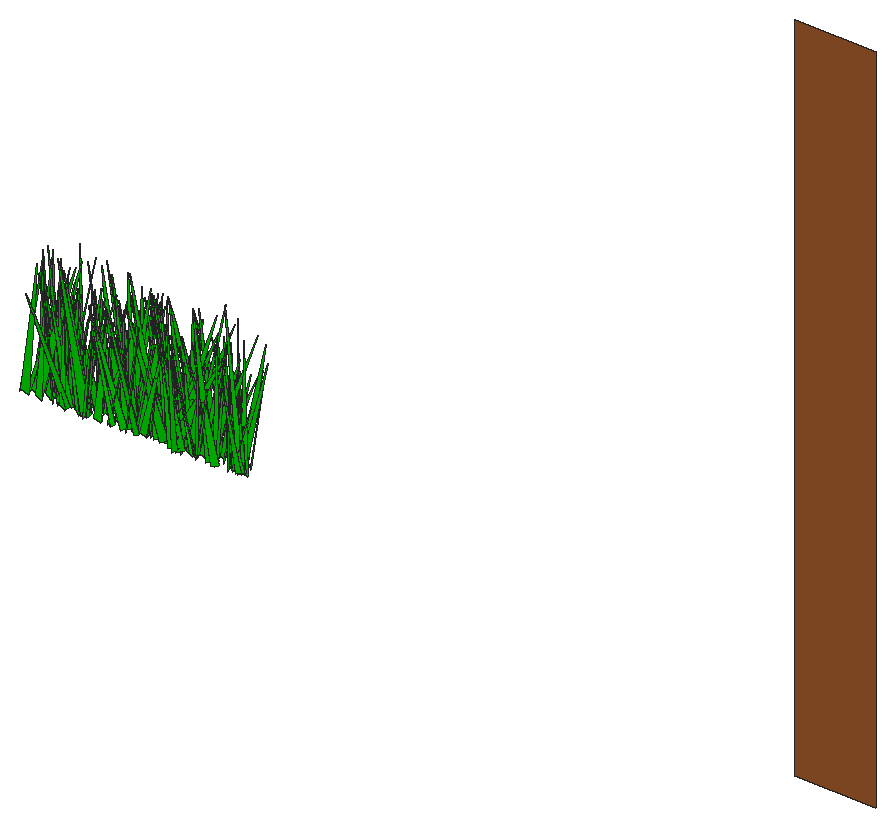
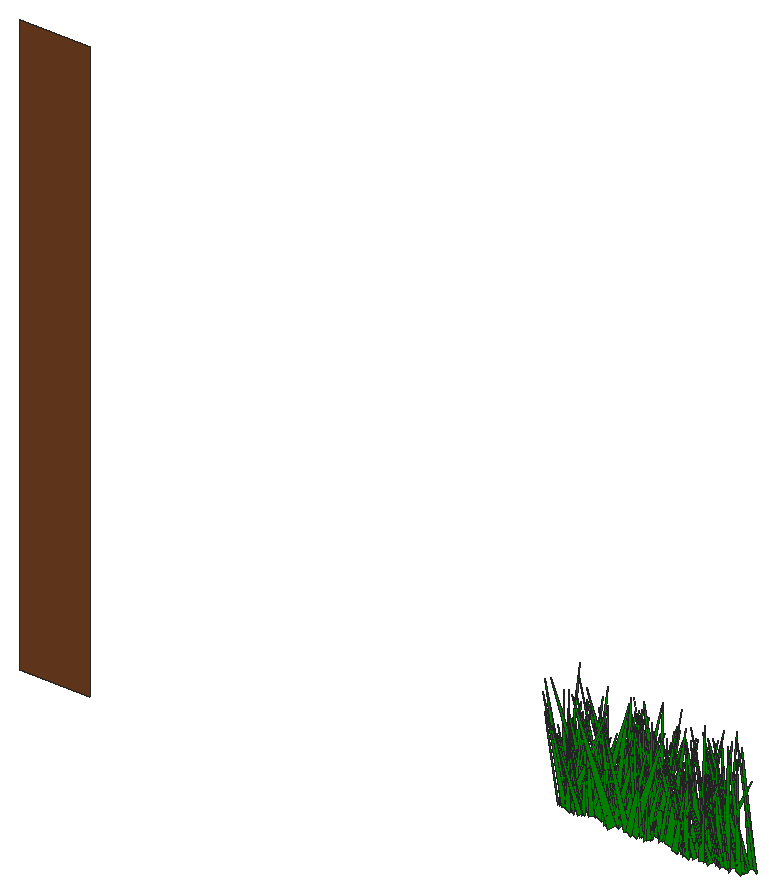
# SketchUp Ruby script. Lengths in inches.
U = 1.inch
M = Sketchup.active_model
def pt(a) = Geom::Point3d.new(a.map { |v| v * U })
def face(e, loops, mat)
  f = e.add_face(loops[0].map { |a| pt(a) })
  loops[1..].each { |l| e.add_face(l.map { |a| pt(a) }).erase! }
  f.material = f.back_material = mat if mat
  f
end
# faces: each face lists its corners as indices into pts; further lists are holes
def faces(e, pts, list, mat = nil) = list.each { |f| face(e, (f[0].is_a?(Array) ? f : [f]).map { |l| l.map { |i| pts[i] } }, mat) }
# xy, xz, yz: faces in a plane at the given z, y or x. An outline is a flat list of corners, or four numbers for a rectangle; further outlines are holes
def ring(l) = l.size == 4 ? [[l[0], l[1]], [l[2], l[1]], [l[2], l[3]], [l[0], l[3]]] : l.each_slice(2).to_a
def flat(e, list, mat, &to3) = list.each { |f| face(e, (f[0].is_a?(Array) ? f : [f]).map { |l| ring(l).map { |u, v| to3.(u, v) } }, mat) }
def xy(e, z, list, mat = nil) = flat(e, list, mat) { |x, y| [x, y, z] }
def xz(e, y, list, mat = nil) = flat(e, list, mat) { |x, z| [x, y, z] }
def yz(e, x, list, mat = nil) = flat(e, list, mat) { |y, z| [x, y, z] }
def lines(e, pts, list) = list.each { |a, b| e.add_line(pt(pts[a]), pt(pts[b])) }
# prism: a flat outline (further loops are holes) pulled along v
def prism(e, loops, v, mat = nil)
  f = face(e, loops, mat); d = Geom::Vector3d.new(v.map { |x| x * U })
  f.pushpull(f.normal.samedirection?(d) ? d.length : -d.length)
end
def box(e, o, s, mat = nil) = prism(e, [[o, [o[0] + s[0], o[1], o[2]], [o[0] + s[0], o[1] + s[1], o[2]], [o[0], o[1] + s[1], o[2]]]], [0, 0, s[2]], mat)
def at(x, y, z, deg = 0) = Geom::Transformation.translation(pt([x, y, z])) * Geom::Transformation.rotation(ORIGIN, Z_AXIS, deg.degrees)
def axes(o, x, y, z) = Geom::Transformation.new([*x, 0, *y, 0, *z, 0, *pt(o).to_a, 1])
def part(name) = M.definitions.add(name)
# library, detail: a bought-in or finely detailed component or shape, given as its bounding box
def library(name, o, s) = part(name).tap { |d| box(d.entities, o, s) }
def detail(e, o, s) = box(e.add_group.entities, o, s)
def put(e, d, t, mat = nil) = e.add_instance(d, t).tap { |i| i.material = mat if mat }
def group(e, t, mat = nil) = e.add_group.tap { |g| g.transformation = t; g.material = mat if mat }.entities
root = M.entities
M.materials.add("[Color G06]").color = [0, 204, 0]
M.materials.add("[Wood Cherry Original]").color = [152, 86, 42]
c1 = part("fur_instance\#9")
p = [[0.8125,0,1.79],[0.67,-0.02,1.48],[0,-0.11,0],[0,0.11,0]]
faces(c1.entities,p,[[0,1,2,3]])
xz(root,22.6875,[[185.87,-6,195.87,78.0625]],"[Wood Cherry Original]")
put(root,c1,axes([90.75,21.5,4.28],[5.77654,-0.14101,0.91321],[-0.79836,-0.77931,-2.54261],[-0.87092,-0.22088,8.38784]),"[Color G06]")
put(root,c1,axes([91.5,21.11,4.28],[-0.85789,-0.67798,2.43897],[-4.9466,0.17029,1.5514],[1.35385,0.1926,7.21388]),"[Color G06]")
put(root,c1,axes([92.05,22.86,4.28],[4.30362,-0.42153,1.03224],[-2.7064,-0.59104,-2.52169],[-1.51342,-0.14175,7.44478]),"[Color G06]")
put(root,c1,axes([91.67,22.66,4.28],[3.5957,0.50169,2.911],[4.0744,-0.47178,-1.9017],[-0.36938,-0.3203,7.36048]),"[Color G06]")
put(root,c1,axes([91.55,21.75,4.28],[2.8548,-0.23429,0.35859],[-1.68592,-0.38392,1.16542],[0.19559,0.11045,4.81171]),"[Color G06]")
put(root,c1,axes([91.41,22.63,4.28],[1.66363,-0.54431,1.55744],[-3.82077,-0.16089,2.65711],[1.31311,0.22147,5.7582]),"[Color G06]")
put(root,c1,axes([93.62,23.0625,4.28],[2.95021,0.59501,2.05008],[4.18656,-0.4476,1.46576],[-1.60043,-0.07405,7.61338]),"[Color G06]")
put(root,c1,axes([93.37,21.03,4.28],[-2.48687,0.47237,0.88273],[3.16901,0.3543,-1.83675],[1.33462,0.03892,6.00611]),"[Color G06]")
put(root,c1,axes([93.03,23.36,4.28],[3.67722,0.16366,1.47306],[1.36394,-0.51239,-1.06592],[-0.69897,-0.13885,5.66969]),"[Color G06]")
put(root,c1,axes([94.99,22.44,4.28],[2.40548,0.60816,3.86018],[4.65114,-0.42329,1.18649],[-2.0145,-0.25111,7.34877]),"[Color G06]")
put(root,c1,axes([95.05,21.68,4.28],[-5.30945,-0.29589,0.88904],[-1.57502,0.66086,4.2551],[1.54127,-0.34395,7.41089]),"[Color G06]")
put(root,c1,axes([96.86,21.02,4.28],[-2.6796,-0.51717,0.40223],[-3.33295,0.31352,-3.28936],[-1.64886,0.20671,5.99533]),"[Color G06]")
put(root,c1,axes([94.67,21.47,4.28],[-5.49241,-0.26482,2.42432],[-1.39314,0.77838,2.71725],[2.07291,-0.17856,8.2497]),"[Color G06]")
put(root,c1,axes([93.99,22.08,4.28],[-1.99993,0.51449,1.73232],[3.62755,0.31264,-1.31169],[1.34059,-0.07845,6.13365]),"[Color G06]")
put(root,c1,axes([95.77,22.24,4.28],[-2.5522,-0.46766,1.16482],[-3.42643,0.33168,-1.47246],[-0.3384,0.1687,6.12422]),"[Color G06]")
put(root,c1,axes([94.23,22.27,4.28],[4.72584,-0.36883,1.81363],[-2.47397,-0.67914,-1.46574],[-1.53225,-0.04102,7.96028]),"[Color G06]")
put(root,c1,axes([93,22.03,4.28],[5.5632,0.02966,0.84503],[0.32456,-0.76274,-1.69724],[-0.5095,-0.162,8.14575]),"[Color G06]")
put(root,c1,axes([92.73,21.54,4.28],[0.23879,0.84781,0.23545],[5.63904,-0.02263,-3.41524],[2.27837,-0.03285,8.42815]),"[Color G06]")
put(root,c1,axes([95.39,21.62,4.28],[1.01177,0.41255,0.83542],[2.83124,-0.15834,1.32309],[-1.02439,-0.03016,4.48194]),"[Color G06]")
put(root,c1,axes([95.86,22,4.28],[-1.95234,-0.44736,1.56321],[-3.37127,0.2514,-1.14033],[-0.14419,0.17941,5.49584]),"[Color G06]")
put(root,c1,axes([94.6875,22.85,4.28],[-0.7828,-0.54813,1.32894],[-3.90732,0.13417,1.21584],[0.98729,0.09638,5.86556]),"[Color G06]")
put(root,c1,axes([95.08,22.09,4.28],[-1.57413,-0.63877,0.32971],[-4.49138,0.2213,1.35276],[0.9273,-0.01248,7.11177]),"[Color G06]")
put(root,c1,axes([93.19,22.5,4.28],[4.14305,-0.58159,0.9089],[-4.17709,-0.5507,2.05211],[0.56258,0.19415,8.54321]),"[Color G06]")
put(root,c1,axes([94.57,23.22,4.28],[3.89882,-0.06393,1.08738],[-0.23994,-0.5332,-1.67911],[-0.82578,-0.14689,5.62182]),"[Color G06]")
put(root,c1,axes([94.38,22.97,4.28],[1.63974,0.41098,0.78915],[2.93482,-0.20398,-1.41863],[0.59323,-0.12688,4.83699]),"[Color G06]")
put(root,c1,axes([93.91,21.81,4.28],[3.96904,0.41017,1.72029],[3.15696,-0.50677,-2.38975],[0.10255,-0.27436,6.98602]),"[Color G06]")
put(root,c1,axes([96.8,21.45,4.28],[0.69713,-0.54996,2.04055],[-3.85603,-0.15872,-1.97145],[-1.59673,0.14319,5.65188]),"[Color G06]")
put(root,c1,axes([95.68,22.6875,4.28],[3.10862,-0.54074,0.2911],[-3.66621,-0.42025,-2.22436],[-1.27835,-0.10969,7.08715]),"[Color G06]")
put(root,c1,axes([95.14,21.79,4.28],[3.60552,0.26626,0.17684],[1.81242,-0.48668,1.63319],[-0.61237,0.12728,5.87493]),"[Color G06]")
put(root,c1,axes([97.55,21.89,4.28],[-3.77417,-0.07772,0.3548],[-0.60132,0.50603,-1.55379],[0.07378,0.14835,5.48617]),"[Color G06]")
put(root,c1,axes([96.29,21,4.28],[-2.28635,0.37225,0.68504],[2.52764,0.32329,-1.33671],[0.97338,0.03487,5.08019]),"[Color G06]")
put(root,c1,axes([96.07,21.88,4.28],[4.17016,0.23642,3.64369],[2.46523,-0.60237,-1.81246],[-1.65552,-0.30146,6.47931]),"[Color G06]")
put(root,c1,axes([98.48,22.83,4.28],[-3.87533,0.32316,0.44032],[2.29533,0.51192,1.96591],[-0.43465,-0.17793,6.45591]),"[Color G06]")
put(root,c1,axes([98.08,21.75,4.28],[-2.41642,-0.35127,1.73454],[-2.72173,0.25903,-2.44367],[-0.53362,0.26951,4.60936]),"[Color G06]")
put(root,c1,axes([95.79,21.54,4.28],[4.56046,0.05114,1.57379],[0.14042,-0.63966,1.47892],[-1.10616,0.12964,6.6761]),"[Color G06]")
put(root,c1,axes([98.1,21.02,4.28],[-5.77826,0.16689,1.15458],[0.82313,0.75849,-3.39286],[1.16259,0.29246,8.14059]),"[Color G06]")
put(root,c1,axes([97.07,23.3125,4.28],[-4.63476,-0.47558,2.68947],[-3.33424,0.69134,1.20873],[1.93721,0.05208,8.51496]),"[Color G06]")
put(root,c1,axes([96.26,22.58,4.28],[4.00094,-0.30757,0.85195],[-2.01319,-0.55254,-1.79593],[-1.06625,-0.11086,6.58774]),"[Color G06]")
put(root,c1,axes([97.47,23.04,4.28],[-3.57017,0.20912,1.35117],[1.33057,0.51008,-1.21563],[1.13837,0.05965,5.65841]),"[Color G06]")
put(root,c1,axes([95.41,22.79,4.28],[5.93196,0.04099,1.18941],[0.13923,-0.82025,1.69625],[-0.83687,0.15409,8.71305]),"[Color G06]")
put(root,c1,axes([97.05,21.67,4.28],[-3.46113,-0.08099,2.9321],[-1.24498,0.50998,-1.66452],[1.62362,0.2184,4.97413]),"[Color G06]")
put(root,c1,axes([98.54,21.35,4.28],[-0.72305,0.61105,0.0274],[4.20016,0.0959,1.89676],[-1.24932,-0.03123,6.36099]),"[Color G06]")
put(root,c1,axes([96.31,22.03,4.28],[-1.13673,-0.69873,0.26377],[-4.79227,0.15883,2.20058],[1.47415,-0.02246,7.35719]),"[Color G06]")
put(root,c1,axes([96.43,22.34,4.28],[0.49402,0.46154,1.39836],[3.34126,-0.03311,-1.38129],[0.81638,-0.14377,4.8071]),"[Color G06]")
put(root,c1,axes([99.05,21.16,4.28],[-0.59035,-0.76245,2.82892],[-5.55675,0.00076,-2.56681],[-1.61278,0.27648,7.80832]),"[Color G06]")
put(root,c1,axes([98.99,21.59,4.28],[-3.01552,-0.60874,1.18417],[-4.43297,0.40785,-1.13111],[-0.18389,0.15062,7.8487]),"[Color G06]")
put(root,c1,axes([95.875,23.2,4.28],[2.44685,-0.42447,0.36241],[-2.77277,-0.29069,2.70589],[1.27921,0.18183,5.17198]),"[Color G06]")
put(root,c1,axes([98.33,22.22,4.28],[2.68568,-0.19433,1.77851],[-1.18125,-0.40867,-1.14502],[-1.40099,-0.02796,4.3748]),"[Color G06]")
put(root,c1,axes([99.62,22.4,4.28],[-0.25277,-0.63232,1.00105],[-4.33838,0.00281,-2.24306],[-1.4795,0.09979,6.40636]),"[Color G06]")
put(root,c1,axes([97.12,21.94,4.28],[4.90886,-0.07684,1.04347],[-0.33022,-0.66448,-2.15131],[-0.82588,-0.19106,7.06235]),"[Color G06]")
put(root,c1,axes([98.19,22.32,4.28],[3.70001,-0.25399,0.30462],[-1.51512,-0.4599,-2.94254],[-1.03129,-0.23559,5.41594]),"[Color G06]")
put(root,c1,axes([99.27,22.82,4.28],[-4.538,0.06593,2.24994],[-0.21901,0.60668,-3.02884],[1.56263,0.27649,6.10951]),"[Color G06]")
put(root,c1,axes([97.43,22.57,4.28],[0.66849,-0.71747,0.74363],[-5.00809,-0.07256,2.01395],[1.2805,0.09076,7.48843]),"[Color G06]")
put(root,c1,axes([100.18,23.13,4.28],[-5.34957,-0.12737,1.85022],[-1.21256,0.73349,-2.03088],[0.94685,0.21971,7.85267]),"[Color G06]")
put(root,c1,axes([96.58,23.17,4.28],[4.12741,0.41844,0.37135],[2.90292,-0.53738,-2.5114],[0.79952,-0.20898,7.20137]),"[Color G06]")
put(root,c1,axes([98.97,23.68,4.28],[3.40014,-0.54772,0.17661],[-3.71936,-0.45559,-2.36084],[-1.26828,-0.13233,7.39685]),"[Color G06]")
put(root,c1,axes([99.11,20.75,4.28],[2.52773,0.26966,0.00061],[1.67322,-0.30503,2.38404],[-0.96951,0.17663,4.11607]),"[Color G06]")
put(root,c1,axes([98.64,21.1,4.28],[3.14584,0.13771,0.55299],[0.7665,-0.41007,1.9902],[-0.72427,0.16414,4.50815]),"[Color G06]")
put(root,c1,axes([100.9,23.29,4.28],[-0.77756,0.5008,0.46133],[3.33548,0.08327,2.17401],[-1.36669,-0.0817,5.04332]),"[Color G06]")
put(root,c1,axes([99.19,23.61,4.28],[-2.11674,-0.44261,0.09561],[-2.88561,0.27271,2.31928],[1.32365,-0.1133,5.20901]),"[Color G06]")
put(root,c1,axes([97.97,23.39,4.28],[2.72019,-0.31903,0.10639],[-2.23299,-0.36648,1.29026],[0.50294,0.09835,5.1532]),"[Color G06]")
put(root,c1,axes([99.45,20.97,4.28],[4.09278,0.30576,1.66908],[2.01331,-0.58986,1.38515],[-1.41473,0.04511,6.79984]),"[Color G06]")
put(root,c1,axes([100.78,23.55,4.28],[0.73569,0.39292,2.65367],[3.05903,-0.17999,1.16711],[-1.31704,-0.19857,4.19312]),"[Color G06]")
put(root,c1,axes([99.1,21.15,4.28],[4.78776,0.15133,1.21649],[0.8068,-0.65236,2.22979],[-1.09057,0.18176,6.99016]),"[Color G06]")
put(root,c1,axes([101.72,21.58,4.28],[-5.60921,-0.06219,1.84379],[-0.98837,0.69708,-4.01538],[0.86253,0.39431,7.38932]),"[Color G06]")
put(root,c1,axes([100.61,21.55,4.28],[-3.88482,-0.2991,1.4639],[-1.85702,0.5503,1.90799],[1.45311,-0.09637,6.35198]),"[Color G06]")
put(root,c1,axes([99.73,22.86,4.28],[3.3637,0.09772,0.65952],[0.59521,-0.46425,1.12054],[-0.57575,0.09094,5.01148]),"[Color G06]")
put(root,c1,axes([101.47,22.2,4.28],[-3.75884,0.30307,0.43313],[1.97956,0.50356,-2.10171],[0.94282,0.151,6.13959]),"[Color G06]")
put(root,c1,axes([98.66,22.9,4.28],[4.41575,-0.30311,0.24717],[-2.1412,-0.59328,1.86971],[0.40931,0.16645,7.11435]),"[Color G06]")
put(root,c1,axes([100.27,22.6,4.28],[3.58173,-0.18823,0.94745],[-1.16112,-0.49631,-1.52183],[-0.9358,-0.10463,5.51455]),"[Color G06]")
put(root,c1,axes([100.47,21.14,4.28],[-1.23098,0.50944,0.8012],[3.54211,0.18518,-1.36921],[1.04279,-0.02763,5.5967]),"[Color G06]")
put(root,c1,axes([102.36,21.15,4.28],[-3.99869,0.24662,0.82912],[1.84302,0.54861,1.10879],[0.1975,-0.12621,6.44006]),"[Color G06]")
put(root,c1,axes([102.25,22.81,4.28],[-2.78447,0.64926,2.27555],[4.89413,0.35827,1.6345],[-0.20943,-0.25977,7.94172]),"[Color G06]")
put(root,c1,axes([100.02,23.19,4.28],[4.53127,-0.02874,1.2027],[-0.36923,-0.62714,1.38557],[-0.74412,0.13615,6.63621]),"[Color G06]")
put(root,c1,axes([103.71,21.27,4.28],[-3.29078,0.47201,0.24779],[3.23559,0.42801,2.327],[-1.00794,-0.16708,6.66093]),"[Color G06]")
put(root,c1,axes([103.54,22.59,4.28],[-5.62166,0.28434,0.264],[1.92141,0.75797,-2.3886],[0.70521,0.2015,8.61253]),"[Color G06]")
put(root,c1,axes([103.62,22.34,4.28],[-5.93887,0.15013,2.41364],[1.49191,0.81681,2.3635],[1.24152,-0.26338,8.70563]),"[Color G06]")
put(root,c1,axes([101.89,22.43,4.28],[3.48564,-0.2179,0.67018],[-1.31656,-0.46515,-2.07747],[-0.95363,-0.15426,5.31768]),"[Color G06]")
put(root,c1,axes([100.54,22.71,4.28],[3.34871,-0.50722,0.07556],[-3.56433,-0.45557,1.5456],[0.72737,0.10275,7.22598]),"[Color G06]")
put(root,c1,axes([104.25,22.26,4.28],[-2.71609,0.70538,0.58674],[5.04808,0.36947,1.17329],[-0.50928,-0.09968,8.5006]),"[Color G06]")
put(root,c1,axes([102.83,22.07,4.28],[-2.07521,-0.55611,1.33459],[-3.90415,0.31105,1.32859],[1.20802,0.04994,6.58642]),"[Color G06]")
put(root,c1,axes([103.98,21.5,4.28],[-0.84514,0.68379,1.25872],[4.94265,0.10173,1.06453],[-0.57033,-0.13165,7.36034]),"[Color G06]")
put(root,c1,axes([101.74,21.23,4.28],[3.82994,0.07741,0.40104],[0.59875,-0.52315,-1.1724],[-0.14724,-0.11377,5.66387]),"[Color G06]")
put(root,c1,axes([105.08,21.74,4.28],[-3.32748,0.21683,0.2617],[1.5205,0.43448,1.83103],[-0.36972,-0.16469,5.17502]),"[Color G06]")
put(root,c1,axes([105.28,21.21,4.28],[-3.44352,-0.46664,0.45012],[-3.32448,0.46449,-1.49436],[-0.48694,0.12881,7.0192]),"[Color G06]")
put(root,c1,axes([102.43,22.09,4.28],[1.02485,0.45329,1.03198],[3.23223,-0.11255,-1.49098],[0.77223,-0.13049,4.87103]),"[Color G06]")
put(root,c1,axes([105.2,22.44,4.28],[-4.56428,-0.17649,0.82389],[-1.34536,0.62819,-1.19032],[0.3094,0.12799,6.97826]),"[Color G06]")
put(root,c1,axes([104.41,21.66,4.28],[-3.25418,-0.36918,0.25807],[-2.58026,0.44925,1.14983],[0.61761,-0.06835,6.16358]),"[Color G06]")
put(root,c1,axes([104.5,21.97,4.28],[0.21627,0.53048,2.04318],[3.93382,-0.07156,1.20418],[-0.93045,-0.17924,5.56605]),"[Color G06]")
put(root,c1,axes([104.19,22.18,4.28],[4.61762,-0.53455,2.35077],[-3.47436,-0.67845,-2.47786],[-2.25785,-0.04924,8.62059]),"[Color G06]")
put(root,c1,axes([105.41,22.84,4.28],[-1.85134,0.44299,0.3253],[3.11172,0.24424,1.35012],[-0.67562,-0.08896,5.32692]),"[Color G06]")
put(root,c1,axes([103.25,21.93,4.28],[1.78588,0.56567,2.03284],[4.27637,-0.22943,-1.05777],[0.13656,-0.21296,6.53941]),"[Color G06]")
put(root,c1,axes([102.6,22.21,4.28],[0.90521,0.4156,1.37204],[2.76057,-0.04477,-2.51033],[1.45081,-0.17411,3.92054]),"[Color G06]")
put(root,c1,axes([106.91,23.36,4.28],[-1.82719,0.69746,1.17457],[4.76649,0.19768,3.07884],[-1.70723,-0.19456,7.33886]),"[Color G06]")
put(root,c1,axes([105.19,22.51,4.28],[2.35284,0.74683,0.29483],[5.13097,-0.32258,2.40074],[-1.54777,0.06593,8.40679]),"[Color G06]")
put(root,c1,axes([106.33,22.71,4.28],[-1.49669,0.67581,1.00724],[4.78692,0.18187,1.87062],[-1.01368,-0.13897,7.34648]),"[Color G06]")
put(root,c1,axes([104.94,23.6875,4.28],[-2.48855,-0.3085,0.29167],[-1.95633,0.32384,2.06278],[1.05131,-0.12763,4.52892]),"[Color G06]")
put(root,c1,axes([104.06,21.23,4.28],[4.31095,-0.0424,1.41402],[-0.03698,-0.59376,-1.79333],[-0.99307,-0.16194,6.20509]),"[Color G06]")
put(root,c1,axes([103.23,22.42,4.28],[2.47724,-0.64614,1.73081],[-4.70287,-0.29824,2.2456],[0.83364,0.23762,7.525]),"[Color G06]")
put(root,c1,axes([103.35,22.31,4.28],[1.57242,-0.83964,0.22921],[-5.91575,-0.21113,1.8083],[1.133,0.06294,9.12362]),"[Color G06]")
put(root,c1,axes([103.57,22.25,4.28],[4.22147,0.15003,0.65039],[1.15858,-0.5582,-2.0061],[-0.06803,-0.19653,6.19424]),"[Color G06]")
put(root,c1,axes([105.68,23.02,4.28],[-2.90846,0.24562,1.07087],[1.56404,0.41284,-1.38898],[1.08154,0.0635,4.88843]),"[Color G06]")
put(root,c1,axes([105.9,22.08,4.28],[-3.2766,0.31174,0.49044],[2.01784,0.43998,-2.01334],[1.01678,0.13144,5.57603]),"[Color G06]")
put(root,c1,axes([104.73,23.1875,4.28],[4.63274,-0.24169,2.64309],[-2.13363,-0.65511,1.47219],[-1.25661,0.2213,7.2446]),"[Color G06]")
put(root,c1,axes([107.6,21.83,4.28],[-3.67082,0.66559,1.71898],[4.89317,0.47951,2.01241],[-0.40323,-0.24045,8.77161]),"[Color G06]")
put(root,c1,axes([105.9375,22.57,4.28],[-3.29205,0.55935,1.70057],[3.92293,0.48401,-1.32465],[1.41263,-0.04058,7.64168]),"[Color G06]")
put(root,c1,axes([104.79,23.05,4.28],[3.90352,-0.19623,0.37174],[-1.31689,-0.53314,-1.43967],[-0.55485,-0.11515,6.0322]),"[Color G06]")
put(root,c1,axes([105.77,23.27,4.28],[-1.9977,0.35233,0.12695],[2.28266,0.25787,-1.97804],[1.08657,0.10603,4.38884]),"[Color G06]")
put(root,c1,axes([107.42,23.55,4.28],[-2.22581,-0.56206,1.10563],[-4.05347,0.2847,-1.60223],[-0.60271,0.16101,6.69255]),"[Color G06]")
put(root,c1,axes([108.24,21.78,4.28],[-2.64068,-0.61799,0.34001],[-4.24442,0.34096,-2.4431],[-1.29518,0.14264,7.31302]),"[Color G06]")
put(root,c1,axes([107.47,22.33,4.28],[-0.99387,-0.54386,1.47537],[-3.84936,0.08733,-2.09428],[-1.1696,0.17473,5.63899]),"[Color G06]")
put(root,c1,axes([104.93,22.5625,4.28],[0.76983,0.56382,0.57625],[3.9573,-0.0918,-1.49152],[0.91468,-0.07738,5.968]),"[Color G06]")
put(root,c1,axes([105.68,22.78,4.28],[2.51448,0.35994,0.03228],[2.52459,-0.3438,1.09183],[-0.53805,0.06897,5.27386]),"[Color G06]")
put(root,c1,axes([106.97,23.14,4.28],[1.01949,-0.37499,0.33914],[-2.41005,-0.14173,-1.81877],[-1.21431,-0.03353,3.89446]),"[Color G06]")
put(root,c1,axes([106.35,22.37,4.28],[-2.67716,-0.03934,2.26842],[-0.72984,0.4056,-1.11593],[1.36036,0.14018,3.86551]),"[Color G06]")
put(root,c1,axes([106.62,23.02,4.28],[-3.97112,0.55544,0.23082],[3.61674,0.51483,-3.32462],[1.67607,0.20508,7.72099]),"[Color G06]")
put(root,c1,axes([105.13,21.28,4.28],[5.718,0.24624,0.9242],[1.62693,-0.79131,1.73465],[-0.92391,0.1305,8.77437]),"[Color G06]")
put(root,c1,axes([105.625,21.7,4.28],[-0.03124,0.77147,0.32132],[5.38324,0.01124,-1.93065],[1.29391,-0.02813,8.04013]),"[Color G06]")
put(root,c1,axes([106.57,22.95,4.28],[-4.07006,0.49115,0.20175],[2.81641,0.47045,-4.6488],[2.11935,0.31803,6.56525]),"[Color G06]")
put(root,c1,axes([108.77,22.09,4.28],[-2.42265,0.37507,0.98388],[2.61016,0.26858,2.59488],[-0.92462,-0.22454,4.74732]),"[Color G06]")
put(root,c1,axes([108.4,22.52,4.28],[-0.7439,-0.7605,0.79046],[-5.33833,0.08382,-1.95861],[-1.23501,0.09578,7.98994]),"[Color G06]")
put(root,c1,axes([105.81,21.59,4.28],[1.88802,-0.42338,0.48029],[-3.01623,-0.25048,1.12031],[0.47319,0.09263,5.22483]),"[Color G06]")
put(root,c1,axes([106.61,21.82,4.28],[3.13466,-0.07005,1.04138],[-0.26137,-0.42799,-1.54991],[-0.81826,-0.13165,4.48448]),"[Color G06]")
put(root,c1,axes([107.68,22.19,4.28],[-2.76319,0.35216,0.13286],[2.3937,0.37065,-1.65506],[0.80998,0.10603,5.3444]),"[Color G06]")
put(root,c1,axes([108.86,21.86,4.28],[-2.52328,0.6519,1.88487],[4.8419,0.33813,1.04489],[-0.03852,-0.201,7.87077]),"[Color G06]")
put(root,c1,axes([107.58,22.05,4.28],[-1.43452,0.48194,1.10385],[3.35117,0.22079,-1.34558],[1.12239,-0.04327,5.42838]),"[Color G06]")
put(root,c1,axes([109.8,22.96,4.28],[-2.50027,0.4998,0.7008],[3.54391,0.32327,1.75845],[-0.71214,-0.14605,6.29029]),"[Color G06]")
put(root,c1,axes([109.8,21.94,4.28],[-1.68973,0.4649,0.41417],[3.21161,0.2133,1.76393],[-0.93675,-0.10731,5.30046]),"[Color G06]")
put(root,c1,axes([109.54,22.26,4.28],[-5.04548,0.18788,2.17546],[1.72149,0.69037,2.06934],[0.98513,-0.24414,7.52577]),"[Color G06]")
put(root,c1,axes([109.64,22.15,4.28],[-1.68157,0.34738,1.07054],[2.51251,0.18917,1.76433],[-0.6373,-0.17081,4.13106]),"[Color G06]")
put(root,c1,axes([110.95,21.32,4.28],[-5.23921,-0.27237,1.4908],[-2.18929,0.62801,-4.00582],[-0.13079,0.39837,7.33418]),"[Color G06]")
put(root,c1,axes([108.85,21.88,4.28],[2.14652,-0.73921,1.12002],[-5.26662,-0.31178,-1.09216],[-0.96207,0.05749,8.47766]),"[Color G06]")
put(root,c1,axes([110.13,21.32,4.28],[-4.78761,-0.21857,0.85015],[-1.47943,0.66805,1.11998],[0.76922,-0.07553,7.44538]),"[Color G06]")
put(root,c1,axes([110.76,21.2,4.28],[-0.13354,-0.67219,4.30524],[-5.23587,-0.13033,-2.70034],[-2.0298,0.38041,6.68228]),"[Color G06]")
put(root,c1,axes([109.47,21.27,4.28],[-2.89359,0.30366,2.27197],[2.56386,0.40116,1.13453],[0.69258,-0.21636,5.29231]),"[Color G06]")
put(root,c1,axes([110.17,21.3,4.28],[-5.31763,0.23255,1.04072],[1.47484,0.73282,-1.97735],[1.04441,0.14918,8.09114]),"[Color G06]")
put(root,c1,axes([109.38,21.9375,4.28],[-3.78856,-0.07485,1.77236],[-0.10286,0.52453,2.05344],[1.29761,-0.17695,5.33744]),"[Color G06]")
put(root,c1,axes([110.21,21.65,4.28],[-2.37776,-0.47332,2.91387],[-3.91438,0.28863,-1.74907],[0.01379,0.31708,5.94188]),"[Color G06]")
put(root,c1,axes([107.87,23.34,4.28],[2.00341,0.5971,0.34499],[4.20537,-0.26663,-1.53956],[0.83867,-0.0894,6.89576]),"[Color G06]")
put(root,c1,axes([110.72,22.32,4.28],[1.18265,-0.69392,3.13031],[-5.09666,-0.24215,-1.86514],[-1.78161,0.23208,7.41354]),"[Color G06]")
put(root,c1,axes([110.25,20.91,4.28],[3.21911,0.46818,2.20116],[2.95865,-0.49314,2.38402],[-2.16519,0.02222,6.53026]),"[Color G06]")
put(root,c1,axes([110.32,21.56,4.28],[-3.99252,0.0524,1.45031],[-0.04968,0.52631,-2.48977],[1.03941,0.22642,5.45186]),"[Color G06]")
put(root,c1,axes([109.16,22.51,4.28],[-3.50904,0.61378,0.53952],[3.53052,0.42849,-4.7052],[2.65326,0.24159,6.97445]),"[Color G06]")
put(root,c1,axes([110.66,21.61,4.28],[-3.44687,-0.02445,1.48784],[0.21567,0.46415,1.99233],[0.98755,-0.18671,4.75797]),"[Color G06]")
put(root,c1,axes([112.43,22.85,4.28],[-1.78128,-0.77361,1.27299],[-5.38915,0.20091,-2.81884],[-1.56848,0.18825,8.23961]),"[Color G06]")
put(root,c1,axes([111.24,23.03,4.28],[-3.43089,-0.10037,0.35251],[-0.55643,0.43749,2.21273],[0.51391,-0.19639,4.74917]),"[Color G06]")
put(root,c1,axes([111.1,22.77,4.28],[-3.82727,-0.26771,0.50118],[-1.64746,0.49947,2.54628],[1.04121,-0.19377,5.87107]),"[Color G06]")
put(root,c1,axes([110.79,23.62,4.28],[-2.90609,-0.28647,0.51668],[-1.82663,0.39018,1.9018],[1.00161,-0.11959,4.96739]),"[Color G06]")
put(root,c1,axes([111.98,21.32,4.28],[-4.37964,0.16222,0.31856],[1.10615,0.6022,-1.25626],[0.41844,0.10591,6.65513]),"[Color G06]")
put(root,c1,axes([110.26,22.77,4.28],[-1.56776,0.60722,2.1803],[4.40444,0.25968,-1.2334],[1.30037,-0.14746,6.80626]),"[Color G06]")
put(root,c1,axes([111.13,22.3,4.28],[1.84773,-0.46718,0.00114],[-3.17704,-0.24437,-1.81442],[-1.0634,-0.08167,5.42278]),"[Color G06]")
put(root,c1,axes([111.34,22.34,4.28],[1.46911,0.72173,0.86633],[5.1379,-0.21458,1.0736],[-0.8519,-0.04955,7.96904]),"[Color G06]")
put(root,c1,axes([110.36,22.84,4.28],[3.36753,-0.44092,2.91877],[-3.67075,-0.45205,1.61564],[-0.5808,0.30054,6.7122]),"[Color G06]")
put(root,c1,axes([112.65,21.17,4.28],[-3.55736,-0.05933,0.0823],[-0.40395,0.48482,1.14568],[0.14445,-0.10526,5.23062]),"[Color G06]")
put(root,c1,axes([111.39,23.09,4.28],[-2.06094,-0.33353,0.44895],[-2.23832,0.28523,1.38974],[0.89499,-0.0547,4.50948]),"[Color G06]")
put(root,c1,axes([110.76,23.24,4.28],[-3.72328,-0.3795,2.41339],[-2.00786,0.55205,3.05288],[2.44593,-0.12451,6.17985]),"[Color G06]")
put(root,c1,axes([113.24,22.67,4.28],[-2.0899,0.53083,1.18648],[3.74798,0.24148,2.33578],[-1.03622,-0.19715,6.05554]),"[Color G06]")
put(root,c1,axes([109.3125,22.08,4.28],[1.75504,0.81465,0.88087],[5.52042,-0.1997,-3.35243],[2.00054,-0.16361,8.47815]),"[Color G06]")
put(root,c1,axes([109.26,22.28,4.28],[2.0008,-0.71349,1.28942],[-4.75146,-0.20011,3.74883],[2.08513,0.22863,7.30531]),"[Color G06]")
put(root,c1,axes([110.64,22.22,4.28],[2.89052,0.41873,0.80637],[3.04243,-0.3879,-1.22219],[0.22717,-0.13289,6.10826]),"[Color G06]")
put(root,c1,axes([111.65,21.58,4.28],[-0.20393,0.49303,1.66627],[3.56236,0.06916,-1.37694],[1.02625,-0.14211,5.11079]),"[Color G06]")
put(root,c1,axes([112.68,21.32,4.28],[3.14477,0.2604,1.74754],[1.61399,-0.4657,1.48384],[-1.4998,0.04485,5.26104]),"[Color G06]")
put(root,c1,axes([109.31,22.02,4.28],[2.28685,-0.68318,0.77],[-4.14218,-0.22379,4.67033],[2.66658,0.23827,6.5944]),"[Color G06]")
put(root,c1,axes([109.74,23.6,4.28],[2.90997,-0.72619,0.47988],[-4.80795,-0.35331,3.70796],[2.02646,0.20455,8.10834]),"[Color G06]")
put(root,c1,axes([114.11,22.59,4.28],[2.26952,0.57929,4.10369],[4.42715,-0.42736,1.46098],[-2.27973,-0.25321,6.92247]),"[Color G06]")
put(root,c1,axes([114.67,21.85,4.28],[-1.71663,-0.48785,0.23671],[-3.34707,0.22131,-1.82424],[-1.03042,0.09387,5.53125]),"[Color G06]")
put(root,c1,axes([114.23,21.53,4.28],[2.15126,-0.7034,2.53667],[-4.9047,-0.36113,-2.21215],[-2.0663,0.12487,7.89188]),"[Color G06]")
put(root,c1,axes([111.27,22.52,4.28],[6.113,-0.1482,1.0185],[-1.14485,-0.84876,1.16168],[-0.53217,0.12358,9.20032]),"[Color G06]")
put(root,c1,axes([116.07,23.24,4.28],[-4.39744,-0.52448,0.80391],[-3.64234,0.54928,-3.33878],[-1.08122,0.28273,7.97791]),"[Color G06]")
put(root,c1,axes([113.19,22.99,4.28],[-2.0371,0.43693,0.57101],[2.94962,0.28607,-1.64029],[1.12399,0.04116,5.33939]),"[Color G06]")
put(root,c1,axes([112.76,21.43,4.28],[3.01193,-0.09626,0.55522],[-0.52283,-0.39991,-1.62919],[-0.58409,-0.1384,4.32135]),"[Color G06]")
put(root,c1,axes([115.02,21.22,4.28],[-1.96425,0.59057,0.34167],[4.16034,0.26146,1.51133],[-0.82454,-0.08763,6.81168]),"[Color G06]")
put(root,c1,axes([116.4,23.25,4.28],[-2.81202,0.56439,0.32654],[3.7085,0.34328,3.17877],[-1.63594,-0.19196,6.64462]),"[Color G06]")
put(root,c1,axes([114.25,23.15,4.28],[3.5765,0.32994,2.38157],[2.02306,-0.5446,1.8808],[-2.01118,0.03893,6.12705]),"[Color G06]")
put(root,c1,axes([112.875,21.98,4.28],[4.83436,-0.27563,1.16396],[-2.09454,-0.66353,1.38259],[-0.3555,0.16117,7.6825]),"[Color G06]")
put(root,c1,axes([114.15,22.44,4.28],[4.9017,-0.46149,0.12566],[-2.82357,-0.59373,-4.45504],[-1.72831,-0.33886,7.63462]),"[Color G06]")
put(root,c1,axes([116.29,22.67,4.28],[-4.60553,0.12057,1.36962],[1.07911,0.62744,1.76057],[0.65027,-0.18732,6.77864]),"[Color G06]")
put(root,c1,axes([114.34,23.31,4.28],[2.92025,0.05269,0.62909],[0.2252,-0.39145,1.43112],[-0.51887,0.12664,4.16172]),"[Color G06]")
put(root,c1,axes([115.62,23.45,4.28],[3.68972,-0.39646,0.85815],[-1.99735,-0.44124,-4.23396],[-2.10323,-0.27649,5.52629]),"[Color G06]")
put(root,c1,axes([113.5625,22.6,4.28],[1.13742,-0.63294,0.49632],[-4.28205,-0.13267,2.48529],[1.54161,0.09849,6.53707]),"[Color G06]")
put(root,c1,axes([115.1,21.34,4.28],[3.97766,0.3852,0.70351],[2.40798,-0.52815,2.80831],[-1.4332,0.18172,6.67089]),"[Color G06]")
put(root,c1,axes([114.67,22.89,4.28],[2.32217,0.33959,1.44174],[2.61819,-0.3064,-1.12921],[-0.07988,-0.1705,4.90083]),"[Color G06]")
put(root,c1,axes([116.33,22.11,4.28],[1.41921,0.62786,1.79825],[4.48515,-0.23166,1.3846],[-1.26648,-0.11683,6.91857]),"[Color G06]")
put(root,c1,axes([116.59,23.4,4.28],[-1.68042,0.30664,1.17753],[2.33193,0.21236,1.08086],[-0.13569,-0.14793,3.9926]),"[Color G06]")
put(root,c1,axes([117.33,22.35,4.28],[-2.16335,-0.4117,1.87908],[-3.14932,0.23181,-2.26469],[-0.61594,0.26078,4.97962]),"[Color G06]")
put(root,c1,axes([115.31,22.24,4.28],[2.60716,0.06889,0.70871],[0.62402,-0.34621,-1.26185],[-0.282,-0.12918,3.75983]),"[Color G06]")
put(root,c1,axes([116.44,23.17,4.28],[4.82454,0.19441,3.2465],[0.92616,-0.72974,1.94547],[-2.40921,0.10878,7.24913]),"[Color G06]")
put(root,c1,axes([116.1,23.64,4.28],[2.4251,-0.33715,0.22577],[-2.23399,-0.32278,-1.76898],[-0.93686,-0.10304,4.80262]),"[Color G06]")
put(root,c1,axes([117.09,21.78,4.28],[-0.0819,-0.5979,0.84321],[-4.25759,-0.00266,-1.14007],[-0.75864,0.07945,6.30724]),"[Color G06]")
put(root,c1,axes([113.375,22.73,4.28],[4.87903,0.51247,1.32545],[3.5949,-0.5664,-4.40238],[1.17024,-0.39671,7.99769]),"[Color G06]")
put(root,c1,axes([116.45,22.59,4.28],[1.9354,-0.46997,0.24851],[-3.2561,-0.26712,-1.38634],[-0.88553,-0.04495,5.64072]),"[Color G06]")
put(root,c1,axes([114.4,23.57,4.28],[2.55324,-0.4313,0.22936],[-2.88579,-0.32131,2.3499],[1.12354,0.15486,5.51446]),"[Color G06]")
put(root,c1,axes([116.67,21.22,4.28],[3.28785,0.18867,1.83378],[0.92319,-0.47566,1.92459],[-1.57601,0.11498,4.95297]),"[Color G06]")
put(root,c1,axes([115.35,23.29,4.28],[2.56417,0.35778,1.35385],[2.70695,-0.31785,-1.8029],[0.27555,-0.20682,5.11283]),"[Color G06]")
put(root,c1,axes([117.1,21.63,4.28],[-4.03985,0.3443,1.67166],[2.30399,0.58363,-1.37121],[1.42788,0.03237,6.9421]),"[Color G06]")
put(root,c1,axes([117.75,21.4375,4.28],[-0.32486,-0.42853,1.11933],[-3.03817,0.01306,-1.39511],[-0.88009,0.11308,4.40288]),"[Color G06]")
put(root,c1,axes([117.6,23.1875,4.28],[-3.38753,-0.14222,0.62243],[-0.85142,0.45715,1.64863],[0.69911,-0.1324,5.02382]),"[Color G06]")
put(root,c1,axes([117.99,21.57,4.28],[-5.49512,0.3121,3.0238],[2.64439,0.78045,1.4809],[1.45253,-0.24012,8.74344]),"[Color G06]")
put(root,c1,axes([117.8,22.3125,4.28],[-4.59386,0.01152,2.24239],[-0.38625,0.6413,-2.14608],[1.45214,0.20703,6.523]),"[Color G06]")
put(root,c1,axes([116.875,23.27,4.28],[0.51754,0.54386,1.12054],[3.84175,-0.04182,-1.63186],[1.0071,-0.11996,5.64918]),"[Color G06]")
put(root,c1,axes([118.23,21.67,4.28],[1.35649,-0.32631,0.55957],[-2.21284,-0.19594,-1.14318],[-0.84816,-0.01068,3.87751]),"[Color G06]")
put(root,c1,axes([118.24,21.66,4.28],[-3.14819,0.61649,0.36899],[4.26534,0.43356,-1.92407],[1.18887,0.07699,7.88015]),"[Color G06]")
put(root,c1,axes([116.87,21.5625,4.28],[2.70441,0.1586,0.29967],[1.14543,-0.35923,-1.24984],[0.14779,-0.11813,4.20296]),"[Color G06]")
put(root,c1,axes([117.32,22.71,4.28],[2.44385,-0.59696,0.40069],[-4.2621,-0.33311,1.05608],[0.48303,0.08105,7.29131]),"[Color G06]")
put(root,c1,axes([118.06,23,4.28],[4.03431,0.05667,1.2846],[0.14405,-0.55292,1.79143],[-0.93976,0.15852,5.78926]),"[Color G06]")
put(root,c1,axes([117.26,22.7,4.28],[2.04538,-0.71334,0.5934],[-5.05321,-0.26972,1.66001],[0.88961,0.108,8.06497]),"[Color G06]")
put(root,c1,axes([117.76,21.98,4.28],[3.2421,0.47785,0.65761],[3.44458,-0.44057,-1.15785],[0.2669,-0.11853,6.9548]),"[Color G06]")
